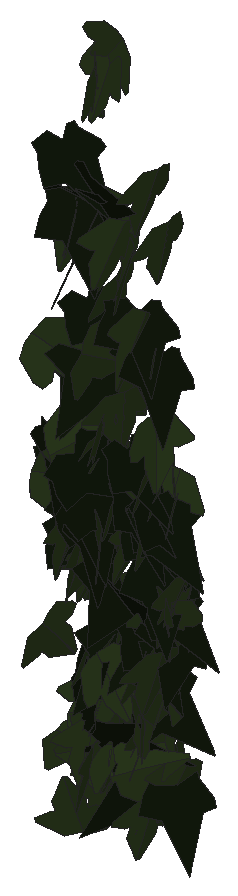
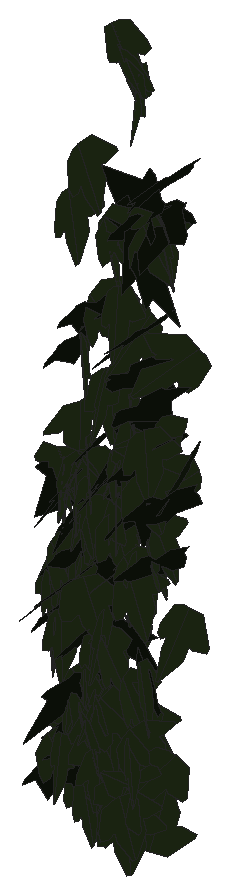
# SketchUp Ruby script. Lengths in inches.
U = 1.inch
M = Sketchup.active_model
def pt(a) = Geom::Point3d.new(a.map { |v| v * U })
def face(e, loops, mat)
  f = e.add_face(loops[0].map { |a| pt(a) })
  loops[1..].each { |l| e.add_face(l.map { |a| pt(a) }).erase! }
  f.material = f.back_material = mat if mat
  f
end
# faces: each face lists its corners as indices into pts; further lists are holes
def faces(e, pts, list, mat = nil) = list.each { |f| face(e, (f[0].is_a?(Array) ? f : [f]).map { |l| l.map { |i| pts[i] } }, mat) }
# xy, xz, yz: faces in a plane at the given z, y or x. An outline is a flat list of corners, or four numbers for a rectangle; further outlines are holes
def ring(l) = l.size == 4 ? [[l[0], l[1]], [l[2], l[1]], [l[2], l[3]], [l[0], l[3]]] : l.each_slice(2).to_a
def flat(e, list, mat, &to3) = list.each { |f| face(e, (f[0].is_a?(Array) ? f : [f]).map { |l| ring(l).map { |u, v| to3.(u, v) } }, mat) }
def xy(e, z, list, mat = nil) = flat(e, list, mat) { |x, y| [x, y, z] }
def xz(e, y, list, mat = nil) = flat(e, list, mat) { |x, z| [x, y, z] }
def yz(e, x, list, mat = nil) = flat(e, list, mat) { |y, z| [x, y, z] }
def lines(e, pts, list) = list.each { |a, b| e.add_line(pt(pts[a]), pt(pts[b])) }
# prism: a flat outline (further loops are holes) pulled along v
def prism(e, loops, v, mat = nil)
  f = face(e, loops, mat); d = Geom::Vector3d.new(v.map { |x| x * U })
  f.pushpull(f.normal.samedirection?(d) ? d.length : -d.length)
end
def box(e, o, s, mat = nil) = prism(e, [[o, [o[0] + s[0], o[1], o[2]], [o[0] + s[0], o[1] + s[1], o[2]], [o[0], o[1] + s[1], o[2]]]], [0, 0, s[2]], mat)
def at(x, y, z, deg = 0) = Geom::Transformation.translation(pt([x, y, z])) * Geom::Transformation.rotation(ORIGIN, Z_AXIS, deg.degrees)
def axes(o, x, y, z) = Geom::Transformation.new([*x, 0, *y, 0, *z, 0, *pt(o).to_a, 1])
def part(name) = M.definitions.add(name)
# library, detail: a bought-in or finely detailed component or shape, given as its bounding box
def library(name, o, s) = part(name).tap { |d| box(d.entities, o, s) }
def detail(e, o, s) = box(e.add_group.entities, o, s)
def put(e, d, t, mat = nil) = e.add_instance(d, t).tap { |i| i.material = mat if mat }
def group(e, t, mat = nil) = e.add_group.tap { |g| g.transformation = t; g.material = mat if mat }.entities
root = M.entities
M.materials.add("efeu1").color = [18, 25, 13]
M.materials.add("efeu2").color = [43, 57, 29]
c1 = part("ivyleaf_9")
p = [[1.54,2.16,1.25],[1.36,2.04,1.19],[-0.21,0.99,0.68],[-0.71,1.11,0.82],[-0.85,0.86,0.67],[-0.8,0.17,0.21],
  [-0.9,-0.01,0.1],[-0.67,-0.16,-0.02],[-0.08,-0.08,-0.05],[-0.03,-0.6,-0.4],[0.65,-0.88,-0.66],[0.83,-0.6,-0.49],
  [1.29,-0.42,-0.43],[1.8125,-0.07,-0.26],[1.21,0.44,0.15]]
faces(c1.entities,p,[[0,1,2,3,4,5,6,7,8,9,10,11,12,13,14]],"efeu1")
c2 = part("ivyleaf_10")
p = [[0,0.5,-0.03],[-0.0625,2.02,-0.43],[-0.19,2.01,-0.46],[-0.54,1.05,-0.29],[-0.52,0.625,-0.18],[-0.83,0.76,-0.28],
  [-1.16,0.64,-0.33],[-1.15,0.33,-0.24],[-0.77,-0.39,0.02],[-0.3,-0.51,0.16],[0.04,-0.48,0.23],[-0.02,2.01,-0.4375],
  [-0.06,2.01,-0.43],[0.04,-0.49,0.23],[0.67,-0.49,0.14],[1.38,0.36,-0.2],[1.375,0.51,-0.24],[0.81,0.65,-0.19],
  [0.62,0.59,-0.15],[0.6,1.09,-0.28],[0.5,1.23,-0.31]]
faces(c2.entities,p,[[0,1,2,3,4,5,6,7,8,9,10],[11,12,0,13,14,15,16,17,18,19,20]],"efeu2")
put(root,c1,axes([516.49,135.94,193.04],[-0.02748,-0.7092,-0.31424],[0.0629,0.31136,-0.70821],[0.77314,-0.05054,0.04644]))
put(root,c2,axes([516.81,136.59,186.14],[-0.31076,-0.50032,0.42625],[0.07365,-0.49503,-0.52735],[0.65314,-0.18223,0.26228]))
put(root,c2,axes([516.75,134.72,188.8],[-0.15574,-0.60785,-0.51435],[0.14813,0.49283,-0.62727],[0.78236,-0.21431,0.01638]))
put(root,c1,axes([516.41,135.62,193.25],[0.09549,-0.5978,0.53452],[0.10415,-0.5245,-0.60519],[0.79514,0.14049,0.01508]))
put(root,c2,axes([516.92,135.77,182.83],[-0.64638,-0.32422,-0.1895],[-0.16144,-0.10068,0.72293],[-0.33906,0.66602,0.01704]))
put(root,c2,axes([516.51,135.84,185.11],[-0.421,-0.35916,-0.51242],[0.46681,0.23102,-0.54546],[0.41672,-0.62164,0.09335]))
put(root,c2,axes([516.84,136.8,185.86],[0.21852,-0.68342,-0.14358],[0.02225,0.15718,-0.7143],[0.69799,0.20895,0.06772]))
put(root,c2,axes([516.89,136.13,194.64],[-0.17798,-0.74343,-0.04971],[0.01508,0.04751,-0.76443],[0.74494,-0.17858,0.0036]))
put(root,c2,axes([516.71,134.77,193.125],[0.08283,0.26282,0.761],[0.12679,0.75121,-0.27324],[-0.79506,0.14717,0.0357]))
put(root,c2,axes([516.99,136.1,187.68],[0.26849,-0.69659,-0.1656],[-0.02645,0.16709,-0.74574],[0.71551,0.26756,0.03457]))
put(root,c2,axes([517.02,136.92,184.08],[-0.31504,-0.63157,0.16688],[0.01674,-0.19302,-0.69889],[0.65303,-0.29974,0.09842]))
put(root,c2,axes([516.98,135.39,191.58],[0.11498,-0.71346,0.22089],[0.08035,-0.21038,-0.72134],[0.74254,0.13324,0.04385]))
put(root,c2,axes([517.14,136.64,183.63],[-0.43886,-0.57309,0.04169],[-0.02208,-0.0356,-0.72181],[0.57418,-0.4394,0.00411]))
put(root,c2,axes([516.63,134.82,196.78],[0.34938,0.37712,0.69187],[0.36493,0.59333,-0.50769],[-0.69838,0.4987,0.08083]))
put(root,c2,axes([517.125,135.9375,193.24],[-0.28243,-0.66214,0.27353],[0.02639,-0.30344,-0.70728],[0.71593,-0.25002,0.13398]))
put(root,c2,axes([517.17,136.34,190.45],[-0.14338,-0.74091,0.11093],[-0.04345,-0.10453,-0.75431],[0.7479,-0.14811,-0.02255]))
put(root,c1,axes([516.74,135.95,191.17],[0.12383,-0.64879,-0.39765],[0.0534,0.4093,-0.65116],[0.75908,0.07704,0.11068]))
put(root,c1,axes([517.02,136.24,195.84],[-0.32694,-0.68562,0.137],[-0.01502,-0.14432,-0.75808],[0.69902,-0.32377,0.04779]))
put(root,c2,axes([517.17,135.1,200.57],[0.52015,-0.60809,-0.19504],[-0.09179,0.17774,-0.79897],[0.63197,0.52631,0.04448]))
put(root,c2,axes([517.17,135.61,200.45],[-0.23533,-0.6787,0.35841],[0.04145,-0.38557,-0.70291],[0.7664,-0.18755,0.14807]))
put(root,c1,axes([517.27,135.73,199.875],[-0.49351,0.41452,-0.46805],[0.36925,-0.28796,-0.64435],[-0.50454,-0.6162,-0.01375]))
put(root,c1,axes([516.75,135.41,202.3],[0.32572,-0.67329,-0.30174],[0.05371,0.3506,-0.72433],[0.73585,0.27244,0.18644]))
put(root,c2,axes([516.99,136.18,184.35],[0.33374,0.32461,-0.59421],[0.33699,0.49497,0.45966],[0.58728,-0.46848,0.07392]))
put(root,c1,axes([517.24,135.19,201.14],[0.67023,0.40751,-0.24645],[-0.30477,0.04008,-0.76257],[-0.36594,0.71298,0.18372]))
put(root,c2,axes([517.19,135.44,191.02],[0.36284,-0.62123,0.21782],[0.1304,-0.17596,-0.71907],[0.64527,0.38489,0.02283]))
put(root,c2,axes([517.4375,136.04,190.72],[-0.06764,-0.69563,0.2869],[-0.02887,-0.28544,-0.69891],[0.75192,-0.07353,-0.00103]))
put(root,c2,axes([517.43,135.64,190.61],[-0.02451,-0.64527,-0.38576],[0.01893,0.38531,-0.64572],[0.75155,-0.03075,0.00369]))
put(root,c2,axes([517.26,136.77,184.26],[-0.68435,0.04444,-0.22898],[0.22455,-0.06655,-0.68402],[-0.06312,-0.71856,0.04919]))
put(root,c1,axes([517.08,135.96,194.13],[0.11764,-0.7227,-0.23839],[0.03701,0.24637,-0.72862],[0.7601,0.09986,0.07237]))
put(root,c2,axes([517.21,134.74,194.1],[0.21257,0.04788,-0.83473],[0.41948,0.73893,0.14921],[0.72325,-0.44265,0.15879]))
put(root,c2,axes([518.02,135.14,185.69],[0.39497,-0.17944,-0.69683],[-0.65472,0.24014,-0.43294],[0.2985,0.76413,-0.02757]))
put(root,c2,axes([517.74,135.39,185.82],[-0.40221,-0.60764,0.20664],[-0.04017,-0.21955,-0.7238],[0.64055,-0.39531,0.08436]))
put(root,c2,axes([517.61,135.92,187],[0.21279,-0.68285,0.183],[0.06302,-0.17203,-0.71519],[0.70413,0.22176,0.0087]))
put(root,c1,axes([517.4,135.3125,200.84],[-0.13883,-0.73324,-0.31717],[0.05951,0.31154,-0.74627],[0.79668,-0.15104,0.00047]))
put(root,c1,axes([517.42,135.75,192.29],[0.03808,-0.75422,-0.13087],[0.00084,0.13107,-0.75514],[0.76549,0.03738,0.00734]))
put(root,c1,axes([517.72,135.69,196.32],[-0.47079,-0.62643,0.13661],[-0.0387,-0.14141,-0.7818],[0.63998,-0.46937,0.05322]))
put(root,c1,axes([517.34,135.36,186.59],[-0.12471,0.33391,0.7135],[0.26224,-0.66359,0.35639],[0.74284,0.29033,-0.00603]))
put(root,c1,axes([517.27,135.76,197.8],[0.34895,-0.64737,-0.28217],[0.07696,0.34773,-0.70259],[0.70199,0.28368,0.21729]))
put(root,c2,axes([517.68,135.41,185.23],[0.33159,-0.62278,0.27121],[0.11551,-0.24571,-0.70544],[0.66938,0.3509,-0.01262]))
put(root,c2,axes([517.72,135.64,200.84],[0.79188,0.13106,-0.06373],[-0.08719,0.14394,-0.7874],[-0.11677,0.78129,0.15576]))
put(root,c2,axes([517.92,136.1,191.82],[-0.18853,-0.70896,0.17471],[-0.03003,-0.17276,-0.73345],[0.72955,-0.19032,0.01496]))
put(root,c2,axes([517.88,135.49,194.25],[-0.04127,-0.73984,-0.2799],[0.02309,0.27904,-0.74096],[0.79068,-0.04676,0.00703]))
put(root,c1,axes([517.48,135.63,191.46],[0.15172,-0.70872,0.27536],[0.06882,-0.26683,-0.7247],[0.75721,0.16626,0.01069]))
put(root,c2,axes([517.94,136.24,186.48],[-0.18352,-0.59789,0.55946],[-0.00109,-0.57316,-0.61289],[0.81882,-0.13476,0.12457]))
put(root,c2,axes([517.92,135.97,198.48],[0.01023,-0.72779,-0.29579],[0.01114,0.29592,-0.72772],[0.78552,0.00528,0.01417]))
put(root,c2,axes([517.95,136.16,185.36],[-0.02896,-0.72983,0.18529],[-0.02967,-0.18417,-0.73008],[0.7524,-0.03535,-0.02165]))
put(root,c2,axes([517.86,135.16,204.72],[0.32834,-0.67979,-0.3174],[0.06264,0.37009,-0.72785],[0.74762,0.26754,0.20038]))
put(root,c2,axes([517.92,136.38,188.3],[0.16619,-0.70962,0.2174],[0.04093,-0.21368,-0.72877],[0.74104,0.17094,-0.00851]))
put(root,c1,axes([517.28,135.53,201.0625],[0.56,-0.05485,-0.58043],[0.57793,0.15828,0.54263],[0.07682,-0.79085,0.14886]))
put(root,c2,axes([517.94,135.97,193.66],[0.14504,-0.72586,0.23756],[0.07589,-0.22691,-0.73966],[0.75997,0.16119,0.02852]))
put(root,c2,axes([518.04,135.2,194.88],[0.37567,-0.66326,-0.23099],[-0.05192,0.23501,-0.75926],[0.70041,0.37317,0.06761]))
put(root,c2,axes([518.37,136.1,185.15],[-0.59171,-0.00433,0.43275],[-0.43004,-0.07642,-0.58877],[0.04859,-0.72908,0.05914]))
put(root,c2,axes([517.97,136.6,185.14],[-0.24559,-0.68107,-0.07656],[0.15936,0.02235,-0.71002],[0.66657,-0.25627,0.14154]))
put(root,c2,axes([518.11,135.73,192.57],[0.25208,-0.59286,-0.41994],[-0.08586,0.41707,-0.64035],[0.72143,0.2568,0.07052]))
put(root,c1,axes([517.66,134.98,192.88],[0.076,-0.21616,-0.78369],[0.13114,0.78005,-0.20244],[0.8023,-0.10703,0.10733]))
put(root,c1,axes([517.76,134.66,194.08],[0.13207,-0.23624,-0.7395],[-0.04279,0.74676,-0.2462],[0.77513,0.08148,0.11241]))
put(root,c2,axes([518.2,135.57,193.64],[0.19249,-0.14738,-0.75254],[-0.13809,0.75655,-0.18349],[0.7543,0.17612,0.15845]))
put(root,c2,axes([518.17,136.45,185.4],[-0.68712,-0.24609,0.07687],[-0.02658,-0.15006,-0.71789],[0.25644,-0.67492,0.13158]))
put(root,c2,axes([518.24,134.85,191.84],[0.46268,-0.51593,-0.37367],[-0.10425,0.39428,-0.67347],[0.62845,0.44525,0.16339]))
put(root,c2,axes([518.1,134.69,197.09],[-0.05353,-0.46642,-0.73818],[0.2057,0.71201,-0.4648],[0.84861,-0.20201,0.0661]))
put(root,c2,axes([518.15,136.27,188.91],[0.14602,-0.66038,-0.36155],[0.10023,0.38206,-0.65736],[0.74617,0.07792,0.15905]))
put(root,c2,axes([518.51,135.14,205.79],[0.63375,-0.1704,-0.49947],[-0.4121,0.32779,-0.63472],[0.32966,0.73733,0.16674]))
put(root,c1,axes([518.47,135.74,188.47],[-0.69703,-0.32432,-0.00813],[0.00635,0.00563,-0.76879],[0.32436,-0.69706,-0.00243]))
put(root,c2,axes([518.26,136.22,192.21],[-0.7471,0.08307,-0.09765],[0.09512,-0.02795,-0.7515],[-0.08595,-0.75293,0.01712]))
put(root,c2,axes([518.22,135.58,185.71],[-0.36124,-0.53791,-0.39888],[0.20113,0.34514,-0.64759],[0.63875,-0.41289,-0.02167]))
put(root,c2,axes([518.26,135.18,205.2],[0.738,-0.35805,-0.05001],[-0.04392,0.02405,-0.82027],[0.35885,0.7393,0.00247]))
put(root,c2,axes([518.29,136.88,186.24],[0.54368,-0.49134,-0.04819],[-0.02589,0.04321,-0.73266],[0.49302,0.5441,0.01466]))
put(root,c2,axes([518.66,136.41,189.78],[-0.64616,-0.24459,0.32201],[-0.28182,-0.16292,-0.68926],[0.28999,-0.70333,0.04768]))
put(root,c2,axes([518.35,136.07,186.71],[0.08108,-0.47044,-0.55535],[0.10612,0.56046,-0.45928],[0.72005,-0.02963,0.13023]))
put(root,c2,axes([518.34,135.98,195.88],[0.20763,-0.65917,-0.37428],[0.10176,0.40879,-0.6635],[0.75115,0.12682,0.19334]))
put(root,c2,axes([518.46,135.39,200.31],[-0.1701,-0.70333,0.36719],[0.03574,-0.38194,-0.71503],[0.7926,-0.13372,0.11105]))
put(root,c2,axes([518.48,136.27,183.81],[0.45144,-0.5573,-0.11008],[-0.05266,0.09895,-0.71689],[0.56562,0.45401,0.02112]))
put(root,c1,axes([518.29,135.66,190.13],[-0.2395,-0.64663,0.41145],[0.06991,-0.44771,-0.66292],[0.76324,-0.1619,0.18983]))
put(root,c2,axes([518.3,135.04,188.05],[0.22032,0.6973,0.28447],[0.0907,0.26967,-0.73126],[-0.74761,0.23821,-0.00488]))
put(root,c2,axes([518.79,136.4,187.12],[0.46192,-0.34658,-0.50755],[-0.41502,0.2924,-0.57737],[0.45331,0.62087,-0.01141]))
put(root,c2,axes([518.57,136.51,183.91],[0.0427,-0.71689,-0.05118],[-0.01049,0.05065,-0.71812],[0.71864,0.04333,-0.00744]))
put(root,c2,axes([518.62,135.39,195.59],[-0.28582,-0.74303,-0.05137],[0.00891,0.0516,-0.79604],[0.74475,-0.28578,-0.01019]))
put(root,c2,axes([518.68,135.95,191.74],[0.06946,-0.67362,0.33681],[0.0204,-0.33643,-0.67707],[0.75285,0.07127,-0.01273]))
put(root,c1,axes([518.24,135.77,189.38],[-0.07507,-0.22955,0.73009],[0.48706,-0.58019,-0.13234],[0.59034,0.44949,0.20203]))
put(root,c2,axes([518.8125,135.94,187.93],[0.07445,-0.66199,-0.38008],[-0.0175,0.3803,-0.6658],[0.76314,0.0733,0.02181]))
put(root,c1,axes([518.22,135.18,185.82],[0.62816,0.17577,0.47658],[0.46556,0.1039,-0.65196],[-0.20315,0.78161,-0.02051]))
put(root,c1,axes([518.89,135.97,184.67],[-0.05246,-0.06216,-0.76835],[0.21274,-0.74139,0.04546],[-0.74092,-0.20847,0.06745]))
put(root,c2,axes([518.84,136.03,192.55],[0.02439,-0.72301,-0.23447],[0.04641,0.23557,-0.72157],[0.75866,0.00883,0.05168]))
put(root,c2,axes([518.82,136.09,186.09],[0.2226,-0.68689,0.17507],[0.04076,-0.17079,-0.72193],[0.70767,0.2259,-0.01349]))
put(root,c2,axes([518.88,135.21,199.76],[0.4289,-0.68381,-0.07997],[-0.03283,0.0738,-0.8071],[0.68768,0.43,0.01134]))
put(root,c2,axes([518.97,135.97,193.3],[-0.47334,-0.61308,0.07744],[0.00363,-0.1003,-0.77191],[0.61794,-0.46903,0.06385]))
put(root,c1,axes([518.66,136.26,188.59],[0.29014,-0.67865,-0.19584],[0.01477,0.21751,-0.73183],[0.70619,0.27428,0.09577]))
put(root,c1,axes([518.68,135.81,192.64],[0.32489,-0.69303,-0.09297],[-0.03188,0.08773,-0.76537],[0.69852,0.32635,0.00831]))
put(root,c2,axes([519.11,136.86,185.21],[0.08906,-0.59947,-0.38097],[-0.02824,0.38066,-0.60559],[0.70972,0.09037,0.02371]))
put(root,c2,axes([519.14,135.83,183.91],[-0.22365,-0.67746,0.1323],[-0.02486,-0.13107,-0.71321],[0.68981,-0.22437,0.01719]))
put(root,c2,axes([518.64,136.5625,186.22],[0.59733,-0.02776,0.42573],[0.42663,0.03741,-0.59616],[0.00085,0.73257,0.04658]))
put(root,c2,axes([519.08,135.72,193.48],[0.33502,-0.66947,-0.18556],[0.00894,0.21014,-0.74204],[0.69466,0.32017,0.09904]))
put(root,c2,axes([519.28,136.33,192.43],[-0.23762,0.60828,-0.39892],[-0.15131,0.36915,0.65302],[0.71151,0.28165,0.00565]))
put(root,c2,axes([519.32,136.34,192.38],[-0.1762,0.49277,-0.55862],[-0.2071,0.519,0.52314],[0.71553,0.27156,0.01385]))
put(root,c2,axes([519,135.5,197.82],[0.0392,-0.65402,0.47141],[0.20562,-0.44825,-0.63899],[0.77955,0.15112,0.14484]))
put(root,c1,axes([518.72,135.54,194.09],[0.36283,-0.64485,-0.2374],[-0.02036,0.25826,-0.73262],[0.68686,0.34829,0.10369]))
put(root,c2,axes([519.18,135.28,186.77],[0.54185,-0.42999,-0.32666],[-0.124,0.35131,-0.66814],[0.52557,0.5262,0.17914]))
put(root,c1,axes([518.86,135.71,197.98],[-0.07915,-0.75082,-0.21288],[0.06014,0.20747,-0.75409],[0.7781,-0.09241,0.03663]))
put(root,c2,axes([519.22,135.59,186.625],[0.01458,0.48083,0.55988],[-0.22846,0.53542,-0.45387],[-0.70175,-0.16432,0.1594]))
put(root,c2,axes([519.13,135.9,196.72],[0.4781,-0.61186,-0.14227],[0.02992,0.20077,-0.76288],[0.62747,0.45664,0.14479]))
put(root,c1,axes([518.88,136.38,186.98],[0.25806,-0.452,-0.59556],[-0.0749,0.61124,-0.49635],[0.7439,0.21834,0.15663]))
put(root,c1,axes([518.93,136.12,192.27],[0.3331,-0.61782,-0.29652],[-0.14031,0.26123,-0.7019],[0.67077,0.36145,0.00043]))
put(root,c2,axes([519.26,135.95,192.81],[0.30095,-0.66609,-0.21565],[0.03567,0.24901,-0.71935],[0.69922,0.27399,0.12951]))
put(root,c2,axes([519.3125,135.58,192.22],[0.14209,-0.57634,-0.52272],[0.00194,0.53162,-0.58563],[0.77807,0.10392,0.09691]))
put(root,c2,axes([518.77,135.34,185.15],[0.11829,0.07052,-0.76771],[0.6698,0.37517,0.13767],[0.38172,-0.68016,-0.00366]))
put(root,c2,axes([519.375,135.6,202.07],[0.00856,-0.79153,0.14294],[0.00437,-0.1429,-0.79157],[0.80432,0.0092,0.00278]))
put(root,c2,axes([519.4,136.45,188.62],[-0.08503,-0.73579,-0.13356],[0.0328,0.13063,-0.74048],[0.74709,-0.08948,0.01731]))
put(root,c2,axes([519.29,135.88,194.75],[0.22559,0.73368,-0.05665],[-0.06208,-0.04006,-0.76611],[-0.73324,0.22911,0.04743]))
put(root,c2,axes([519.625,136.125,192.87],[0.12932,-0.30393,-0.7007],[-0.23493,0.66039,-0.3298],[0.72675,0.26757,0.01807]))
put(root,c2,axes([519.6,136.52,184.92],[-0.12755,-0.659,0.29394],[-0.0351,-0.29248,-0.67095],[0.72073,-0.13087,0.01934]))
put(root,c1,axes([519.32,136.09,190.7],[-0.01686,-0.7712,-0.07628],[0.01215,0.07603,-0.77132],[0.77487,-0.01797,0.01043]))
put(root,c2,axes([519.68,135.71,200.66],[-0.01906,-0.79616,-0.03267],[0.02318,0.03211,-0.79607],[0.79649,-0.01999,0.02239]))
put(root,c2,axes([519.84,136.34,188.43],[0.23894,-0.39122,-0.5916],[-0.24441,0.54061,-0.45622],[0.66582,0.33885,0.04483]))
put(root,c2,axes([519.53,135.75,190.1],[-0.50303,0.50777,-0.23459],[0.10297,-0.22604,-0.71007],[-0.54978,-0.50692,0.08165]))
put(root,c2,axes([519.75,135.79,189.8],[-0.51011,-0.5513,-0.01217],[0.01055,0.00682,-0.75109],[0.55133,-0.51021,0.00311]))
put(root,c1,axes([519.41,135.86,196.88],[0.03804,-0.78879,0.00889],[0.00423,-0.0087,-0.78969],[0.78883,0.03808,0.0038]))
put(root,c2,axes([519.66,136.09,193.32],[0.76365,0.0499,-0.07651],[-0.0759,-0.0118,-0.76525],[-0.05082,0.76739,-0.00679]))
put(root,c1,axes([519.3,136.25,189.83],[0.38517,-0.612,-0.26185],[0.05044,0.32848,-0.69355],[0.66375,0.33018,0.20465]))
put(root,c1,axes([519.39,135.6875,192.78],[0.41415,-0.56825,-0.34605],[-0.10227,0.3484,-0.6945],[0.65741,0.41217,0.10995]))
put(root,c2,axes([519.89,135.21,188.68],[-0.11212,-0.76033,0.12533],[-0.0205,-0.12367,-0.76855],[0.77032,-0.11395,-0.00221]))
put(root,c1,axes([519.6,136.36,184.52],[0.00829,-0.7348,-0.19324],[-0.0179,0.19301,-0.73469],[0.75958,0.01256,-0.0152]))
put(root,c2,axes([519.76,136.48,189.82],[0.1598,-0.7287,0.10141],[0.17244,-0.06379,-0.73008],[0.71522,0.17819,0.15337]))
put(root,c2,axes([519.85,136.06,190.37],[0.15905,-0.7035,0.29125],[0.07295,-0.28208,-0.72121],[0.7579,0.17478,0.0083]))
put(root,c1,axes([519.64,136.31,189],[-0.0732,-0.73059,0.21232],[0.03139,-0.21602,-0.7325],[0.76017,-0.06143,0.0507]))
put(root,c1,axes([519.49,135.54,192.61],[-0.1226,-0.39541,-0.66594],[0.39325,0.54906,-0.39841],[0.66721,-0.39627,0.11246]))
